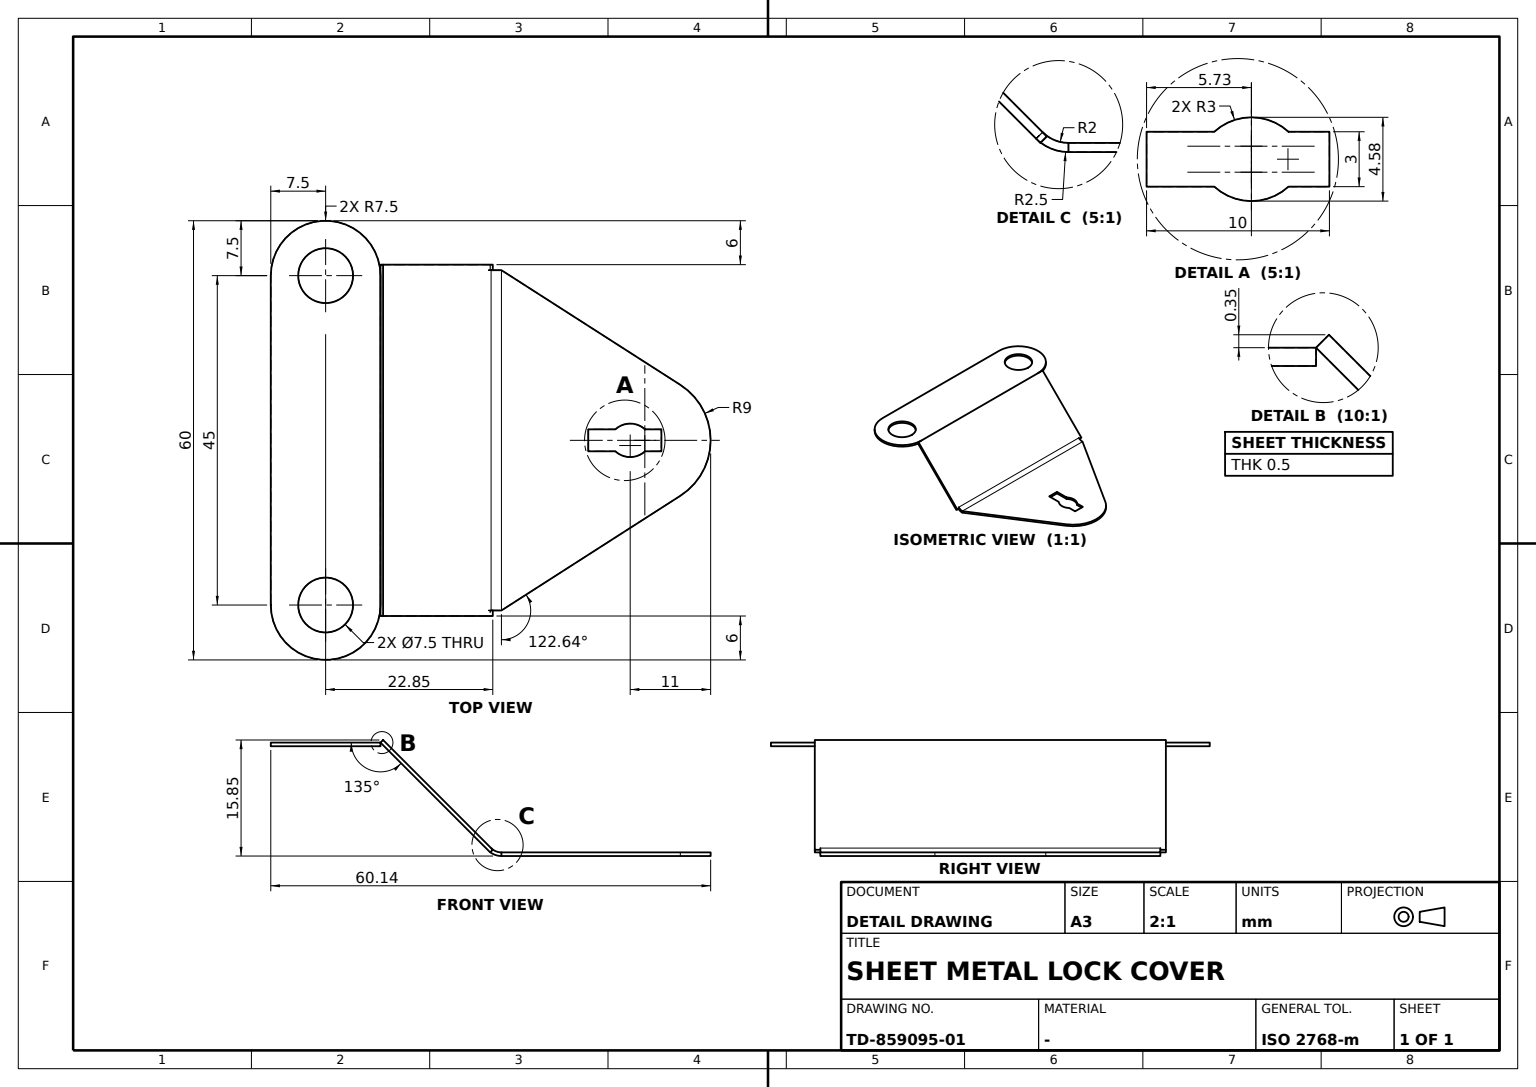
ISO-10303-21;
HEADER;
FILE_DESCRIPTION((''),'2;1');
FILE_NAME('','',(''),(''),'','','');
FILE_SCHEMA(('AUTOMOTIVE_DESIGN'));
ENDSEC;
DATA;
#1=APPLICATION_CONTEXT('');
#2=PRODUCT_CONTEXT('',#1,'mechanical');
#3=PRODUCT('','','',(#2));
#4=PRODUCT_DEFINITION_FORMATION('','',#3);
#5=PRODUCT_DEFINITION_CONTEXT('',#1,'design');
#6=PRODUCT_DEFINITION('','',#4,#5);
#7=PRODUCT_DEFINITION_SHAPE('','',#6);
#8=(LENGTH_UNIT()NAMED_UNIT(*)SI_UNIT(.MILLI.,.METRE.));
#9=(NAMED_UNIT(*)PLANE_ANGLE_UNIT()SI_UNIT($,.RADIAN.));
#10=(NAMED_UNIT(*)SI_UNIT($,.STERADIAN.)SOLID_ANGLE_UNIT());
#11=UNCERTAINTY_MEASURE_WITH_UNIT(LENGTH_MEASURE(0.005),#8,'distance_accuracy_value','');
#12=(GEOMETRIC_REPRESENTATION_CONTEXT(3)GLOBAL_UNCERTAINTY_ASSIGNED_CONTEXT((#11))GLOBAL_UNIT_ASSIGNED_CONTEXT((#8,#9,#10))REPRESENTATION_CONTEXT('',''));
#13=CARTESIAN_POINT('',(3.75,-22.5,0.5));
#14=VERTEX_POINT('',#13);
#15=CARTESIAN_POINT('',(0.,-22.5,0.5));
#16=DIRECTION('',(0.,0.,1.));
#17=DIRECTION('',(1.,0.,0.));
#18=AXIS2_PLACEMENT_3D('',#15,#16,#17);
#19=CIRCLE('',#18,3.75);
#20=EDGE_CURVE('',#14,#14,#19,.T.);
#21=ORIENTED_EDGE('',*,*,#20,.T.);
#22=EDGE_LOOP('',(#21));
#23=FACE_BOUND('',#22,.T.);
#24=CARTESIAN_POINT('',(3.75,-22.5,0.));
#25=VERTEX_POINT('',#24);
#26=CARTESIAN_POINT('',(0.,-22.5,0.));
#27=AXIS2_PLACEMENT_3D('',#26,#16,#17);
#28=CIRCLE('',#27,3.75);
#29=EDGE_CURVE('',#25,#25,#28,.T.);
#30=ORIENTED_EDGE('',*,*,#29,.F.);
#31=EDGE_LOOP('',(#30));
#32=FACE_BOUND('',#31,.T.);
#33=DIRECTION('',(0.,1.,0.));
#34=AXIS2_PLACEMENT_3D('',#15,#16,#33);
#35=CYLINDRICAL_SURFACE('',#34,3.75);
#36=ADVANCED_FACE('',(#23,#32),#35,.F.);
#37=CARTESIAN_POINT('',(3.75,22.5,0.5));
#38=VERTEX_POINT('',#37);
#39=CARTESIAN_POINT('',(0.,22.5,0.5));
#40=AXIS2_PLACEMENT_3D('',#39,#16,#17);
#41=CIRCLE('',#40,3.75);
#42=EDGE_CURVE('',#38,#38,#41,.F.);
#43=ORIENTED_EDGE('',*,*,#42,.T.);
#44=EDGE_LOOP('',(#43));
#45=FACE_BOUND('',#44,.T.);
#46=ORIENTED_EDGE('',*,*,#20,.F.);
#47=EDGE_LOOP('',(#46));
#48=FACE_BOUND('',#47,.T.);
#49=CARTESIAN_POINT('',(-7.5,-22.5,0.5));
#50=VERTEX_POINT('',#49);
#51=CARTESIAN_POINT('',(-7.5,22.5,0.5));
#52=VERTEX_POINT('',#51);
#53=VECTOR('',#33,1000.);
#54=LINE('',#51,#53);
#55=EDGE_CURVE('',#50,#52,#54,.T.);
#56=ORIENTED_EDGE('',*,*,#55,.F.);
#57=CARTESIAN_POINT('',(7.5,-22.5,0.5));
#58=VERTEX_POINT('',#57);
#59=CIRCLE('',#18,7.5);
#60=EDGE_CURVE('',#50,#58,#59,.T.);
#61=ORIENTED_EDGE('',*,*,#60,.T.);
#62=CARTESIAN_POINT('',(7.5,22.5,0.5));
#63=VERTEX_POINT('',#62);
#64=DIRECTION('',(0.,-1.,0.));
#65=VECTOR('',#64,1000.);
#66=LINE('',#57,#65);
#67=EDGE_CURVE('',#63,#58,#66,.T.);
#68=ORIENTED_EDGE('',*,*,#67,.F.);
#69=CIRCLE('',#40,7.5);
#70=EDGE_CURVE('',#63,#52,#69,.T.);
#71=ORIENTED_EDGE('',*,*,#70,.T.);
#72=EDGE_LOOP('',(#56,#61,#68,#71));
#73=FACE_BOUND('',#72,.T.);
#74=CARTESIAN_POINT('',(0.,0.,0.5));
#75=AXIS2_PLACEMENT_3D('',#74,#16,#33);
#76=PLANE('',#75);
#77=ADVANCED_FACE('',(#45,#48,#73),#76,.T.);
#78=ORIENTED_EDGE('',*,*,#42,.F.);
#79=EDGE_LOOP('',(#78));
#80=FACE_BOUND('',#79,.T.);
#81=CARTESIAN_POINT('',(3.75,22.5,0.));
#82=VERTEX_POINT('',#81);
#83=CARTESIAN_POINT('',(0.,22.5,0.));
#84=AXIS2_PLACEMENT_3D('',#83,#16,#17);
#85=CIRCLE('',#84,3.75);
#86=EDGE_CURVE('',#82,#82,#85,.F.);
#87=ORIENTED_EDGE('',*,*,#86,.T.);
#88=EDGE_LOOP('',(#87));
#89=FACE_BOUND('',#88,.T.);
#90=AXIS2_PLACEMENT_3D('',#39,#16,#33);
#91=CYLINDRICAL_SURFACE('',#90,3.75);
#92=ADVANCED_FACE('',(#80,#89),#91,.F.);
#93=CARTESIAN_POINT('',(-7.5,22.5,0.));
#94=VERTEX_POINT('',#93);
#95=VECTOR('',#16,1000.);
#96=LINE('',#93,#95);
#97=EDGE_CURVE('',#52,#94,#96,.F.);
#98=ORIENTED_EDGE('',*,*,#97,.F.);
#99=ORIENTED_EDGE('',*,*,#70,.F.);
#100=CARTESIAN_POINT('',(7.5,22.5,0.));
#101=VERTEX_POINT('',#100);
#102=LINE('',#100,#95);
#103=EDGE_CURVE('',#101,#63,#102,.T.);
#104=ORIENTED_EDGE('',*,*,#103,.F.);
#105=CIRCLE('',#84,7.5);
#106=EDGE_CURVE('',#101,#94,#105,.T.);
#107=ORIENTED_EDGE('',*,*,#106,.T.);
#108=EDGE_LOOP('',(#98,#99,#104,#107));
#109=FACE_BOUND('',#108,.T.);
#110=AXIS2_PLACEMENT_3D('',#83,#16,#33);
#111=CYLINDRICAL_SURFACE('',#110,7.5);
#112=ADVANCED_FACE('',(#109),#111,.T.);
#113=CARTESIAN_POINT('',(-7.5,-22.5,0.));
#114=VERTEX_POINT('',#113);
#115=CARTESIAN_POINT('',(7.5,-22.5,0.));
#116=VERTEX_POINT('',#115);
#117=CIRCLE('',#27,7.5);
#118=EDGE_CURVE('',#114,#116,#117,.T.);
#119=ORIENTED_EDGE('',*,*,#118,.T.);
#120=LINE('',#115,#95);
#121=EDGE_CURVE('',#116,#58,#120,.T.);
#122=ORIENTED_EDGE('',*,*,#121,.T.);
#123=ORIENTED_EDGE('',*,*,#60,.F.);
#124=LINE('',#113,#95);
#125=EDGE_CURVE('',#114,#50,#124,.T.);
#126=ORIENTED_EDGE('',*,*,#125,.F.);
#127=EDGE_LOOP('',(#119,#122,#123,#126));
#128=FACE_BOUND('',#127,.T.);
#129=AXIS2_PLACEMENT_3D('',#26,#16,#33);
#130=CYLINDRICAL_SURFACE('',#129,7.5);
#131=ADVANCED_FACE('',(#128),#130,.T.);
#132=ORIENTED_EDGE('',*,*,#103,.T.);
#133=ORIENTED_EDGE('',*,*,#67,.T.);
#134=ORIENTED_EDGE('',*,*,#121,.F.);
#135=LINE('',#115,#65);
#136=EDGE_CURVE('',#101,#116,#135,.T.);
#137=ORIENTED_EDGE('',*,*,#136,.F.);
#138=EDGE_LOOP('',(#132,#133,#134,#137));
#139=FACE_BOUND('',#138,.T.);
#140=AXIS2_PLACEMENT_3D('',#115,#17,#33);
#141=PLANE('',#140);
#142=ADVANCED_FACE('',(#139),#141,.T.);
#143=ORIENTED_EDGE('',*,*,#97,.T.);
#144=LINE('',#93,#53);
#145=EDGE_CURVE('',#114,#94,#144,.T.);
#146=ORIENTED_EDGE('',*,*,#145,.F.);
#147=ORIENTED_EDGE('',*,*,#125,.T.);
#148=ORIENTED_EDGE('',*,*,#55,.T.);
#149=EDGE_LOOP('',(#143,#146,#147,#148));
#150=FACE_BOUND('',#149,.T.);
#151=DIRECTION('',(-1.,0.,0.));
#152=AXIS2_PLACEMENT_3D('',#93,#151,#64);
#153=PLANE('',#152);
#154=ADVANCED_FACE('',(#150),#153,.T.);
#155=ORIENTED_EDGE('',*,*,#86,.F.);
#156=EDGE_LOOP('',(#155));
#157=FACE_BOUND('',#156,.T.);
#158=ORIENTED_EDGE('',*,*,#29,.T.);
#159=EDGE_LOOP('',(#158));
#160=FACE_BOUND('',#159,.T.);
#161=ORIENTED_EDGE('',*,*,#106,.F.);
#162=ORIENTED_EDGE('',*,*,#136,.T.);
#163=ORIENTED_EDGE('',*,*,#118,.F.);
#164=ORIENTED_EDGE('',*,*,#145,.T.);
#165=EDGE_LOOP('',(#161,#162,#163,#164));
#166=FACE_BOUND('',#165,.T.);
#167=CARTESIAN_POINT('',(0.,0.,0.));
#168=AXIS2_PLACEMENT_3D('',#167,#16,#33);
#169=PLANE('',#168);
#170=ADVANCED_FACE('',(#157,#160,#166),#169,.F.);
#171=CLOSED_SHELL('',(#36,#77,#92,#112,#131,#142,#154,#170));
#172=MANIFOLD_SOLID_BREP('',#171);
#173=CARTESIAN_POINT('',(48.493351,7.578879,-15.));
#174=VERTEX_POINT('',#173);
#175=CARTESIAN_POINT('',(48.493351,7.578879,-14.5));
#176=VERTEX_POINT('',#175);
#177=LINE('',#173,#95);
#178=EDGE_CURVE('',#174,#176,#177,.T.);
#179=ORIENTED_EDGE('',*,*,#178,.F.);
#180=CARTESIAN_POINT('',(24.035534,23.242995,-15.));
#181=VERTEX_POINT('',#180);
#182=CARTESIAN_POINT('',(17.547395,27.398352,-15.));
#183=DIRECTION('',(-0.84209762,0.539325133,0.));
#184=VECTOR('',#183,1000.);
#185=LINE('',#182,#184);
#186=EDGE_CURVE('',#174,#181,#185,.T.);
#187=ORIENTED_EDGE('',*,*,#186,.T.);
#188=CARTESIAN_POINT('',(24.035534,23.242995,-14.5));
#189=VERTEX_POINT('',#188);
#190=LINE('',#180,#95);
#191=EDGE_CURVE('',#181,#189,#190,.T.);
#192=ORIENTED_EDGE('',*,*,#191,.T.);
#193=CARTESIAN_POINT('',(17.547395,27.398352,-14.5));
#194=LINE('',#193,#184);
#195=EDGE_CURVE('',#176,#189,#194,.T.);
#196=ORIENTED_EDGE('',*,*,#195,.F.);
#197=EDGE_LOOP('',(#179,#187,#192,#196));
#198=FACE_BOUND('',#197,.T.);
#199=DIRECTION('',(0.539325133,0.84209762,0.));
#200=AXIS2_PLACEMENT_3D('',#173,#199,#183);
#201=PLANE('',#200);
#202=ADVANCED_FACE('',(#198),#201,.T.);
#203=CARTESIAN_POINT('',(39.611252,-1.5,-15.));
#204=VERTEX_POINT('',#203);
#205=CARTESIAN_POINT('',(39.611252,-1.5,-14.5));
#206=VERTEX_POINT('',#205);
#207=LINE('',#203,#95);
#208=EDGE_CURVE('',#204,#206,#207,.T.);
#209=ORIENTED_EDGE('',*,*,#208,.T.);
#210=CARTESIAN_POINT('',(43.667597,-1.5,-14.5));
#211=VERTEX_POINT('',#210);
#212=CARTESIAN_POINT('',(41.639425,0.710547,-14.5));
#213=AXIS2_PLACEMENT_3D('',#212,#16,#17);
#214=CIRCLE('',#213,3.);
#215=EDGE_CURVE('',#211,#206,#214,.F.);
#216=ORIENTED_EDGE('',*,*,#215,.F.);
#217=CARTESIAN_POINT('',(43.667597,-1.5,-15.));
#218=VERTEX_POINT('',#217);
#219=LINE('',#217,#95);
#220=EDGE_CURVE('',#218,#211,#219,.T.);
#221=ORIENTED_EDGE('',*,*,#220,.F.);
#222=CARTESIAN_POINT('',(41.639425,0.710547,-15.));
#223=AXIS2_PLACEMENT_3D('',#222,#16,#17);
#224=CIRCLE('',#223,3.);
#225=EDGE_CURVE('',#218,#204,#224,.F.);
#226=ORIENTED_EDGE('',*,*,#225,.T.);
#227=EDGE_LOOP('',(#209,#216,#221,#226));
#228=FACE_BOUND('',#227,.T.);
#229=AXIS2_PLACEMENT_3D('',#212,#16,#33);
#230=CYLINDRICAL_SURFACE('',#229,3.);
#231=ADVANCED_FACE('',(#228),#230,.F.);
#232=CARTESIAN_POINT('',(39.611252,1.5,-14.5));
#233=VERTEX_POINT('',#232);
#234=CARTESIAN_POINT('',(35.906857,1.5,-14.5));
#235=VERTEX_POINT('',#234);
#236=CARTESIAN_POINT('',(44.787227,1.5,-14.5));
#237=VECTOR('',#151,1000.);
#238=LINE('',#236,#237);
#239=EDGE_CURVE('',#233,#235,#238,.T.);
#240=ORIENTED_EDGE('',*,*,#239,.T.);
#241=CARTESIAN_POINT('',(35.906857,1.5,-15.));
#242=VERTEX_POINT('',#241);
#243=LINE('',#234,#95);
#244=EDGE_CURVE('',#242,#235,#243,.T.);
#245=ORIENTED_EDGE('',*,*,#244,.F.);
#246=CARTESIAN_POINT('',(39.611252,1.5,-15.));
#247=VERTEX_POINT('',#246);
#248=CARTESIAN_POINT('',(44.787227,1.5,-15.));
#249=LINE('',#248,#237);
#250=EDGE_CURVE('',#247,#242,#249,.T.);
#251=ORIENTED_EDGE('',*,*,#250,.F.);
#252=LINE('',#246,#95);
#253=EDGE_CURVE('',#247,#233,#252,.T.);
#254=ORIENTED_EDGE('',*,*,#253,.T.);
#255=EDGE_LOOP('',(#240,#245,#251,#254));
#256=FACE_BOUND('',#255,.T.);
#257=AXIS2_PLACEMENT_3D('',#236,#64,#17);
#258=PLANE('',#257);
#259=ADVANCED_FACE('',(#256),#258,.T.);
#260=CARTESIAN_POINT('',(24.035534,-23.242995,-14.5));
#261=VERTEX_POINT('',#260);
#262=CARTESIAN_POINT('',(48.493351,-7.578879,-14.5));
#263=VERTEX_POINT('',#262);
#264=CARTESIAN_POINT('',(17.547395,-27.398352,-14.5));
#265=DIRECTION('',(0.84209762,0.539325133,0.));
#266=VECTOR('',#265,1000.);
#267=LINE('',#264,#266);
#268=EDGE_CURVE('',#261,#263,#267,.T.);
#269=ORIENTED_EDGE('',*,*,#268,.T.);
#270=CARTESIAN_POINT('',(43.639425,0.,-14.5));
#271=AXIS2_PLACEMENT_3D('',#270,#16,#17);
#272=CIRCLE('',#271,9.);
#273=EDGE_CURVE('',#263,#176,#272,.T.);
#274=ORIENTED_EDGE('',*,*,#273,.T.);
#275=ORIENTED_EDGE('',*,*,#195,.T.);
#276=CARTESIAN_POINT('',(24.035534,0.,-14.5));
#277=LINE('',#276,#65);
#278=EDGE_CURVE('',#189,#261,#277,.T.);
#279=ORIENTED_EDGE('',*,*,#278,.T.);
#280=EDGE_LOOP('',(#269,#274,#275,#279));
#281=FACE_BOUND('',#280,.T.);
#282=ORIENTED_EDGE('',*,*,#239,.F.);
#283=CARTESIAN_POINT('',(43.667597,1.5,-14.5));
#284=VERTEX_POINT('',#283);
#285=CARTESIAN_POINT('',(41.639425,-0.710547,-14.5));
#286=AXIS2_PLACEMENT_3D('',#285,#16,#17);
#287=CIRCLE('',#286,3.);
#288=EDGE_CURVE('',#233,#284,#287,.F.);
#289=ORIENTED_EDGE('',*,*,#288,.T.);
#290=CARTESIAN_POINT('',(45.906857,1.5,-14.5));
#291=VERTEX_POINT('',#290);
#292=CARTESIAN_POINT('',(0.,1.5,-14.5));
#293=VECTOR('',#17,1000.);
#294=LINE('',#292,#293);
#295=EDGE_CURVE('',#284,#291,#294,.T.);
#296=ORIENTED_EDGE('',*,*,#295,.T.);
#297=CARTESIAN_POINT('',(45.906857,-1.5,-14.5));
#298=VERTEX_POINT('',#297);
#299=CARTESIAN_POINT('',(45.906857,0.,-14.5));
#300=LINE('',#299,#65);
#301=EDGE_CURVE('',#291,#298,#300,.T.);
#302=ORIENTED_EDGE('',*,*,#301,.T.);
#303=CARTESIAN_POINT('',(44.787227,-1.5,-14.5));
#304=LINE('',#303,#237);
#305=EDGE_CURVE('',#298,#211,#304,.T.);
#306=ORIENTED_EDGE('',*,*,#305,.T.);
#307=ORIENTED_EDGE('',*,*,#215,.T.);
#308=CARTESIAN_POINT('',(35.906857,-1.5,-14.5));
#309=VERTEX_POINT('',#308);
#310=EDGE_CURVE('',#206,#309,#304,.T.);
#311=ORIENTED_EDGE('',*,*,#310,.T.);
#312=CARTESIAN_POINT('',(35.906857,0.,-14.5));
#313=LINE('',#312,#53);
#314=EDGE_CURVE('',#309,#235,#313,.T.);
#315=ORIENTED_EDGE('',*,*,#314,.T.);
#316=EDGE_LOOP('',(#282,#289,#296,#302,#306,#307,#311,#315));
#317=FACE_BOUND('',#316,.T.);
#318=CARTESIAN_POINT('',(0.,0.,-14.5));
#319=AXIS2_PLACEMENT_3D('',#318,#16,#33);
#320=PLANE('',#319);
#321=ADVANCED_FACE('',(#281,#317),#320,.T.);
#322=ORIENTED_EDGE('',*,*,#253,.F.);
#323=CARTESIAN_POINT('',(43.667597,1.5,-15.));
#324=VERTEX_POINT('',#323);
#325=CARTESIAN_POINT('',(41.639425,-0.710547,-15.));
#326=AXIS2_PLACEMENT_3D('',#325,#16,#17);
#327=CIRCLE('',#326,3.);
#328=EDGE_CURVE('',#247,#324,#327,.F.);
#329=ORIENTED_EDGE('',*,*,#328,.T.);
#330=LINE('',#323,#95);
#331=EDGE_CURVE('',#324,#284,#330,.T.);
#332=ORIENTED_EDGE('',*,*,#331,.T.);
#333=ORIENTED_EDGE('',*,*,#288,.F.);
#334=EDGE_LOOP('',(#322,#329,#332,#333));
#335=FACE_BOUND('',#334,.T.);
#336=AXIS2_PLACEMENT_3D('',#285,#16,#33);
#337=CYLINDRICAL_SURFACE('',#336,3.);
#338=ADVANCED_FACE('',(#335),#337,.F.);
#339=CARTESIAN_POINT('',(7.5,-24.,0.5));
#340=VERTEX_POINT('',#339);
#341=CARTESIAN_POINT('',(22.5,-24.,-14.5));
#342=VERTEX_POINT('',#341);
#343=CARTESIAN_POINT('',(15.,-24.,-7.));
#344=DIRECTION('',(0.707106781,0.,-0.707106781));
#345=VECTOR('',#344,1000.);
#346=LINE('',#343,#345);
#347=EDGE_CURVE('',#340,#342,#346,.T.);
#348=ORIENTED_EDGE('',*,*,#347,.T.);
#349=CARTESIAN_POINT('',(22.853553,-24.,-14.146447));
#350=VERTEX_POINT('',#349);
#351=CARTESIAN_POINT('',(22.676777,-24.,-14.323223));
#352=DIRECTION('',(-0.707106781,0.,-0.707106781));
#353=VECTOR('',#352,1000.);
#354=LINE('',#351,#353);
#355=EDGE_CURVE('',#350,#342,#354,.T.);
#356=ORIENTED_EDGE('',*,*,#355,.F.);
#357=CARTESIAN_POINT('',(7.853553,-24.,0.853553));
#358=VERTEX_POINT('',#357);
#359=CARTESIAN_POINT('',(15.353553,-24.,-6.646447));
#360=LINE('',#359,#345);
#361=EDGE_CURVE('',#358,#350,#360,.T.);
#362=ORIENTED_EDGE('',*,*,#361,.F.);
#363=CARTESIAN_POINT('',(7.676777,-24.,0.676777));
#364=LINE('',#363,#353);
#365=EDGE_CURVE('',#358,#340,#364,.T.);
#366=ORIENTED_EDGE('',*,*,#365,.T.);
#367=EDGE_LOOP('',(#348,#356,#362,#366));
#368=FACE_BOUND('',#367,.T.);
#369=CARTESIAN_POINT('',(15.176777,-24.,-6.823223));
#370=AXIS2_PLACEMENT_3D('',#369,#33,#17);
#371=PLANE('',#370);
#372=ADVANCED_FACE('',(#368),#371,.F.);
#373=CARTESIAN_POINT('',(24.035534,-23.242995,-15.));
#374=VERTEX_POINT('',#373);
#375=LINE('',#373,#95);
#376=EDGE_CURVE('',#374,#261,#375,.T.);
#377=ORIENTED_EDGE('',*,*,#376,.F.);
#378=CARTESIAN_POINT('',(48.493351,-7.578879,-15.));
#379=VERTEX_POINT('',#378);
#380=CARTESIAN_POINT('',(17.547395,-27.398352,-15.));
#381=LINE('',#380,#266);
#382=EDGE_CURVE('',#374,#379,#381,.T.);
#383=ORIENTED_EDGE('',*,*,#382,.T.);
#384=LINE('',#378,#95);
#385=EDGE_CURVE('',#379,#263,#384,.T.);
#386=ORIENTED_EDGE('',*,*,#385,.T.);
#387=ORIENTED_EDGE('',*,*,#268,.F.);
#388=EDGE_LOOP('',(#377,#383,#386,#387));
#389=FACE_BOUND('',#388,.T.);
#390=CARTESIAN_POINT('',(22.853553,-24.,-15.));
#391=DIRECTION('',(0.539325133,-0.84209762,0.));
#392=AXIS2_PLACEMENT_3D('',#390,#391,#265);
#393=PLANE('',#392);
#394=ADVANCED_FACE('',(#389),#393,.T.);
#395=CARTESIAN_POINT('',(22.267767,-23.242995,-14.267767));
#396=VERTEX_POINT('',#395);
#397=CARTESIAN_POINT('',(22.62132,-23.242995,-13.914214));
#398=VERTEX_POINT('',#397);
#399=DIRECTION('',(0.707106781,0.,0.707106781));
#400=VECTOR('',#399,1000.);
#401=LINE('',#395,#400);
#402=EDGE_CURVE('',#396,#398,#401,.T.);
#403=ORIENTED_EDGE('',*,*,#402,.F.);
#404=CARTESIAN_POINT('',(24.035534,-23.242995,-12.5));
#405=DIRECTION('',(0.,0.,-1.));
#406=AXIS2_PLACEMENT_3D('',#404,#64,#405);
#407=CIRCLE('',#406,2.5);
#408=EDGE_CURVE('',#396,#374,#407,.T.);
#409=ORIENTED_EDGE('',*,*,#408,.T.);
#410=ORIENTED_EDGE('',*,*,#376,.T.);
#411=CIRCLE('',#406,2.);
#412=EDGE_CURVE('',#398,#261,#411,.T.);
#413=ORIENTED_EDGE('',*,*,#412,.F.);
#414=EDGE_LOOP('',(#403,#409,#410,#413));
#415=FACE_BOUND('',#414,.T.);
#416=CARTESIAN_POINT('',(23.878454,-23.242995,-14.5));
#417=CARTESIAN_POINT('',(23.839184,-23.242995,-15.));
#418=CARTESIAN_POINT('',(23.721375,-23.242995,-14.484579));
#419=CARTESIAN_POINT('',(23.642835,-23.242995,-14.980723));
#420=CARTESIAN_POINT('',(23.566314,-23.242995,-14.453735));
#421=CARTESIAN_POINT('',(23.449009,-23.242995,-14.942169));
#422=CARTESIAN_POINT('',(23.264266,-23.242995,-14.362006));
#423=CARTESIAN_POINT('',(23.071449,-23.242995,-14.827508));
#424=CARTESIAN_POINT('',(22.985823,-23.242995,-14.213288));
#425=CARTESIAN_POINT('',(22.723396,-23.242995,-14.64161));
#426=CARTESIAN_POINT('',(22.854369,-23.242995,-14.125453));
#427=CARTESIAN_POINT('',(22.559078,-23.242995,-14.531817));
#428=CARTESIAN_POINT('',(22.732392,-23.242995,-14.025286));
#429=CARTESIAN_POINT('',(22.406607,-23.242995,-14.406607));
#430=B_SPLINE_SURFACE_WITH_KNOTS('',5,1,((#260,#373),(#416,#417),(#418,#419),(#420,#421),(#422,#423),(#424,#425),(#426,#427),(#428,#429),(#397,#395)),.RULED_SURF.,.F.,.F.,.F.,(6,3,6),(2,2),(0.,0.00185,0.0037),(0.,0.00049),.UNSPECIFIED.);
#431=ADVANCED_FACE('',(#415),#430,.T.);
#432=ORIENTED_EDGE('',*,*,#191,.F.);
#433=CARTESIAN_POINT('',(22.267767,23.242995,-14.267767));
#434=VERTEX_POINT('',#433);
#435=CARTESIAN_POINT('',(24.035534,23.242995,-12.5));
#436=AXIS2_PLACEMENT_3D('',#435,#64,#405);
#437=CIRCLE('',#436,2.5);
#438=EDGE_CURVE('',#434,#181,#437,.T.);
#439=ORIENTED_EDGE('',*,*,#438,.F.);
#440=CARTESIAN_POINT('',(22.62132,23.242995,-13.914214));
#441=VERTEX_POINT('',#440);
#442=LINE('',#440,#353);
#443=EDGE_CURVE('',#434,#441,#442,.F.);
#444=ORIENTED_EDGE('',*,*,#443,.T.);
#445=CIRCLE('',#436,2.);
#446=EDGE_CURVE('',#441,#189,#445,.T.);
#447=ORIENTED_EDGE('',*,*,#446,.T.);
#448=EDGE_LOOP('',(#432,#439,#444,#447));
#449=FACE_BOUND('',#448,.T.);
#450=CARTESIAN_POINT('',(23.878454,23.242995,-14.5));
#451=CARTESIAN_POINT('',(23.839184,23.242995,-15.));
#452=CARTESIAN_POINT('',(23.721375,23.242995,-14.484579));
#453=CARTESIAN_POINT('',(23.642835,23.242995,-14.980723));
#454=CARTESIAN_POINT('',(23.566314,23.242995,-14.453735));
#455=CARTESIAN_POINT('',(23.449009,23.242995,-14.942169));
#456=CARTESIAN_POINT('',(23.264266,23.242995,-14.362006));
#457=CARTESIAN_POINT('',(23.071449,23.242995,-14.827508));
#458=CARTESIAN_POINT('',(22.985823,23.242995,-14.213288));
#459=CARTESIAN_POINT('',(22.723396,23.242995,-14.64161));
#460=CARTESIAN_POINT('',(22.854369,23.242995,-14.125453));
#461=CARTESIAN_POINT('',(22.559078,23.242995,-14.531817));
#462=CARTESIAN_POINT('',(22.732392,23.242995,-14.025286));
#463=CARTESIAN_POINT('',(22.406607,23.242995,-14.406607));
#464=B_SPLINE_SURFACE_WITH_KNOTS('',5,1,((#188,#180),(#450,#451),(#452,#453),(#454,#455),(#456,#457),(#458,#459),(#460,#461),(#462,#463),(#440,#433)),.RULED_SURF.,.F.,.F.,.F.,(6,3,6),(2,2),(0.,0.00185,0.0037),(0.,0.00049),.UNSPECIFIED.);
#465=ADVANCED_FACE('',(#449),#464,.F.);
#466=CARTESIAN_POINT('',(22.62132,0.,-13.914214));
#467=LINE('',#466,#65);
#468=EDGE_CURVE('',#441,#398,#467,.T.);
#469=ORIENTED_EDGE('',*,*,#468,.T.);
#470=ORIENTED_EDGE('',*,*,#412,.T.);
#471=ORIENTED_EDGE('',*,*,#278,.F.);
#472=ORIENTED_EDGE('',*,*,#446,.F.);
#473=EDGE_LOOP('',(#469,#470,#471,#472));
#474=FACE_BOUND('',#473,.T.);
#475=CARTESIAN_POINT('',(24.035534,0.,-12.5));
#476=AXIS2_PLACEMENT_3D('',#475,#64,#405);
#477=CYLINDRICAL_SURFACE('',#476,2.);
#478=ADVANCED_FACE('',(#474),#477,.F.);
#479=CARTESIAN_POINT('',(45.906857,-1.5,-15.));
#480=VERTEX_POINT('',#479);
#481=LINE('',#297,#95);
#482=EDGE_CURVE('',#480,#298,#481,.T.);
#483=ORIENTED_EDGE('',*,*,#482,.T.);
#484=ORIENTED_EDGE('',*,*,#301,.F.);
#485=CARTESIAN_POINT('',(45.906857,1.5,-15.));
#486=VERTEX_POINT('',#485);
#487=LINE('',#290,#95);
#488=EDGE_CURVE('',#486,#291,#487,.T.);
#489=ORIENTED_EDGE('',*,*,#488,.F.);
#490=CARTESIAN_POINT('',(45.906857,0.,-15.));
#491=LINE('',#490,#65);
#492=EDGE_CURVE('',#486,#480,#491,.T.);
#493=ORIENTED_EDGE('',*,*,#492,.T.);
#494=EDGE_LOOP('',(#483,#484,#489,#493));
#495=FACE_BOUND('',#494,.T.);
#496=AXIS2_PLACEMENT_3D('',#299,#151,#33);
#497=PLANE('',#496);
#498=ADVANCED_FACE('',(#495),#497,.T.);
#499=ORIENTED_EDGE('',*,*,#438,.T.);
#500=CARTESIAN_POINT('',(24.035534,0.,-15.));
#501=LINE('',#500,#65);
#502=EDGE_CURVE('',#181,#374,#501,.T.);
#503=ORIENTED_EDGE('',*,*,#502,.T.);
#504=ORIENTED_EDGE('',*,*,#408,.F.);
#505=CARTESIAN_POINT('',(22.267767,0.,-14.267767));
#506=LINE('',#505,#65);
#507=EDGE_CURVE('',#434,#396,#506,.T.);
#508=ORIENTED_EDGE('',*,*,#507,.F.);
#509=EDGE_LOOP('',(#499,#503,#504,#508));
#510=FACE_BOUND('',#509,.T.);
#511=CYLINDRICAL_SURFACE('',#476,2.5);
#512=ADVANCED_FACE('',(#510),#511,.T.);
#513=CARTESIAN_POINT('',(7.5,24.,0.5));
#514=VERTEX_POINT('',#513);
#515=CARTESIAN_POINT('',(7.5,0.,0.5));
#516=LINE('',#515,#53);
#517=EDGE_CURVE('',#340,#514,#516,.T.);
#518=ORIENTED_EDGE('',*,*,#517,.T.);
#519=CARTESIAN_POINT('',(22.5,24.,-14.5));
#520=VERTEX_POINT('',#519);
#521=CARTESIAN_POINT('',(15.,24.,-7.));
#522=LINE('',#521,#345);
#523=EDGE_CURVE('',#514,#520,#522,.T.);
#524=ORIENTED_EDGE('',*,*,#523,.T.);
#525=CARTESIAN_POINT('',(22.5,23.242995,-14.5));
#526=VERTEX_POINT('',#525);
#527=CARTESIAN_POINT('',(22.5,0.,-14.5));
#528=LINE('',#527,#53);
#529=EDGE_CURVE('',#526,#520,#528,.T.);
#530=ORIENTED_EDGE('',*,*,#529,.F.);
#531=CARTESIAN_POINT('',(22.383883,23.242995,-14.383883));
#532=LINE('',#531,#345);
#533=EDGE_CURVE('',#434,#526,#532,.T.);
#534=ORIENTED_EDGE('',*,*,#533,.F.);
#535=ORIENTED_EDGE('',*,*,#507,.T.);
#536=CARTESIAN_POINT('',(22.5,-23.242995,-14.5));
#537=VERTEX_POINT('',#536);
#538=CARTESIAN_POINT('',(7.5,-23.242995,0.5));
#539=DIRECTION('',(-0.707106781,0.,0.707106781));
#540=VECTOR('',#539,1000.);
#541=LINE('',#538,#540);
#542=EDGE_CURVE('',#537,#396,#541,.T.);
#543=ORIENTED_EDGE('',*,*,#542,.F.);
#544=EDGE_CURVE('',#342,#537,#528,.T.);
#545=ORIENTED_EDGE('',*,*,#544,.F.);
#546=ORIENTED_EDGE('',*,*,#347,.F.);
#547=EDGE_LOOP('',(#518,#524,#530,#534,#535,#543,#545,#546));
#548=FACE_BOUND('',#547,.T.);
#549=AXIS2_PLACEMENT_3D('',#515,#399,#344);
#550=PLANE('',#549);
#551=ADVANCED_FACE('',(#548),#550,.F.);
#552=ORIENTED_EDGE('',*,*,#443,.F.);
#553=ORIENTED_EDGE('',*,*,#533,.T.);
#554=CARTESIAN_POINT('',(22.853553,23.242995,-14.146447));
#555=VERTEX_POINT('',#554);
#556=LINE('',#525,#400);
#557=EDGE_CURVE('',#526,#555,#556,.T.);
#558=ORIENTED_EDGE('',*,*,#557,.T.);
#559=CARTESIAN_POINT('',(22.737437,23.242995,-14.03033));
#560=LINE('',#559,#345);
#561=EDGE_CURVE('',#441,#555,#560,.T.);
#562=ORIENTED_EDGE('',*,*,#561,.F.);
#563=EDGE_LOOP('',(#552,#553,#558,#562));
#564=FACE_BOUND('',#563,.T.);
#565=AXIS2_PLACEMENT_3D('',#531,#33,#17);
#566=PLANE('',#565);
#567=ADVANCED_FACE('',(#564),#566,.F.);
#568=ORIENTED_EDGE('',*,*,#523,.F.);
#569=CARTESIAN_POINT('',(7.853553,24.,0.853553));
#570=VERTEX_POINT('',#569);
#571=CARTESIAN_POINT('',(7.676777,24.,0.676777));
#572=LINE('',#571,#353);
#573=EDGE_CURVE('',#570,#514,#572,.T.);
#574=ORIENTED_EDGE('',*,*,#573,.F.);
#575=CARTESIAN_POINT('',(22.853553,24.,-14.146447));
#576=VERTEX_POINT('',#575);
#577=CARTESIAN_POINT('',(15.353553,24.,-6.646447));
#578=LINE('',#577,#345);
#579=EDGE_CURVE('',#570,#576,#578,.T.);
#580=ORIENTED_EDGE('',*,*,#579,.T.);
#581=CARTESIAN_POINT('',(22.676777,24.,-14.323223));
#582=LINE('',#581,#353);
#583=EDGE_CURVE('',#576,#520,#582,.T.);
#584=ORIENTED_EDGE('',*,*,#583,.T.);
#585=EDGE_LOOP('',(#568,#574,#580,#584));
#586=FACE_BOUND('',#585,.T.);
#587=CARTESIAN_POINT('',(15.176777,24.,-6.823223));
#588=AXIS2_PLACEMENT_3D('',#587,#33,#17);
#589=PLANE('',#588);
#590=ADVANCED_FACE('',(#586),#589,.T.);
#591=ORIENTED_EDGE('',*,*,#557,.F.);
#592=ORIENTED_EDGE('',*,*,#529,.T.);
#593=ORIENTED_EDGE('',*,*,#583,.F.);
#594=CARTESIAN_POINT('',(22.853553,0.,-14.146447));
#595=LINE('',#594,#53);
#596=EDGE_CURVE('',#555,#576,#595,.T.);
#597=ORIENTED_EDGE('',*,*,#596,.F.);
#598=EDGE_LOOP('',(#591,#592,#593,#597));
#599=FACE_BOUND('',#598,.T.);
#600=CARTESIAN_POINT('',(22.676777,0.,-14.323223));
#601=AXIS2_PLACEMENT_3D('',#600,#539,#399);
#602=PLANE('',#601);
#603=ADVANCED_FACE('',(#599),#602,.F.);
#604=CARTESIAN_POINT('',(44.787227,-1.5,-15.));
#605=LINE('',#604,#237);
#606=EDGE_CURVE('',#480,#218,#605,.T.);
#607=ORIENTED_EDGE('',*,*,#606,.F.);
#608=ORIENTED_EDGE('',*,*,#492,.F.);
#609=CARTESIAN_POINT('',(0.,1.5,-15.));
#610=LINE('',#609,#293);
#611=EDGE_CURVE('',#324,#486,#610,.T.);
#612=ORIENTED_EDGE('',*,*,#611,.F.);
#613=ORIENTED_EDGE('',*,*,#328,.F.);
#614=ORIENTED_EDGE('',*,*,#250,.T.);
#615=CARTESIAN_POINT('',(35.906857,-1.5,-15.));
#616=VERTEX_POINT('',#615);
#617=CARTESIAN_POINT('',(35.906857,0.,-15.));
#618=LINE('',#617,#53);
#619=EDGE_CURVE('',#616,#242,#618,.T.);
#620=ORIENTED_EDGE('',*,*,#619,.F.);
#621=EDGE_CURVE('',#204,#616,#605,.T.);
#622=ORIENTED_EDGE('',*,*,#621,.F.);
#623=ORIENTED_EDGE('',*,*,#225,.F.);
#624=EDGE_LOOP('',(#607,#608,#612,#613,#614,#620,#622,#623));
#625=FACE_BOUND('',#624,.T.);
#626=ORIENTED_EDGE('',*,*,#502,.F.);
#627=ORIENTED_EDGE('',*,*,#186,.F.);
#628=CARTESIAN_POINT('',(43.639425,0.,-15.));
#629=AXIS2_PLACEMENT_3D('',#628,#16,#17);
#630=CIRCLE('',#629,9.);
#631=EDGE_CURVE('',#379,#174,#630,.T.);
#632=ORIENTED_EDGE('',*,*,#631,.F.);
#633=ORIENTED_EDGE('',*,*,#382,.F.);
#634=EDGE_LOOP('',(#626,#627,#632,#633));
#635=FACE_BOUND('',#634,.T.);
#636=CARTESIAN_POINT('',(0.,0.,-15.));
#637=AXIS2_PLACEMENT_3D('',#636,#16,#33);
#638=PLANE('',#637);
#639=ADVANCED_FACE('',(#625,#635),#638,.F.);
#640=ORIENTED_EDGE('',*,*,#314,.F.);
#641=LINE('',#308,#95);
#642=EDGE_CURVE('',#616,#309,#641,.T.);
#643=ORIENTED_EDGE('',*,*,#642,.F.);
#644=ORIENTED_EDGE('',*,*,#619,.T.);
#645=ORIENTED_EDGE('',*,*,#244,.T.);
#646=EDGE_LOOP('',(#640,#643,#644,#645));
#647=FACE_BOUND('',#646,.T.);
#648=AXIS2_PLACEMENT_3D('',#312,#17,#33);
#649=PLANE('',#648);
#650=ADVANCED_FACE('',(#647),#649,.T.);
#651=ORIENTED_EDGE('',*,*,#596,.T.);
#652=ORIENTED_EDGE('',*,*,#579,.F.);
#653=CARTESIAN_POINT('',(7.853553,0.,0.853553));
#654=LINE('',#653,#53);
#655=EDGE_CURVE('',#358,#570,#654,.T.);
#656=ORIENTED_EDGE('',*,*,#655,.F.);
#657=ORIENTED_EDGE('',*,*,#361,.T.);
#658=CARTESIAN_POINT('',(22.853553,-23.242995,-14.146447));
#659=VERTEX_POINT('',#658);
#660=EDGE_CURVE('',#350,#659,#595,.T.);
#661=ORIENTED_EDGE('',*,*,#660,.T.);
#662=CARTESIAN_POINT('',(7.853553,-23.242995,0.853553));
#663=LINE('',#662,#540);
#664=EDGE_CURVE('',#659,#398,#663,.T.);
#665=ORIENTED_EDGE('',*,*,#664,.T.);
#666=ORIENTED_EDGE('',*,*,#468,.F.);
#667=ORIENTED_EDGE('',*,*,#561,.T.);
#668=EDGE_LOOP('',(#651,#652,#656,#657,#661,#665,#666,#667));
#669=FACE_BOUND('',#668,.T.);
#670=AXIS2_PLACEMENT_3D('',#653,#399,#344);
#671=PLANE('',#670);
#672=ADVANCED_FACE('',(#669),#671,.T.);
#673=ORIENTED_EDGE('',*,*,#517,.F.);
#674=ORIENTED_EDGE('',*,*,#365,.F.);
#675=ORIENTED_EDGE('',*,*,#655,.T.);
#676=ORIENTED_EDGE('',*,*,#573,.T.);
#677=EDGE_LOOP('',(#673,#674,#675,#676));
#678=FACE_BOUND('',#677,.T.);
#679=CARTESIAN_POINT('',(7.676777,0.,0.676777));
#680=AXIS2_PLACEMENT_3D('',#679,#539,#399);
#681=PLANE('',#680);
#682=ADVANCED_FACE('',(#678),#681,.T.);
#683=ORIENTED_EDGE('',*,*,#273,.F.);
#684=ORIENTED_EDGE('',*,*,#385,.F.);
#685=ORIENTED_EDGE('',*,*,#631,.T.);
#686=ORIENTED_EDGE('',*,*,#178,.T.);
#687=EDGE_LOOP('',(#683,#684,#685,#686));
#688=FACE_BOUND('',#687,.T.);
#689=AXIS2_PLACEMENT_3D('',#628,#16,#33);
#690=CYLINDRICAL_SURFACE('',#689,9.);
#691=ADVANCED_FACE('',(#688),#690,.T.);
#692=ORIENTED_EDGE('',*,*,#542,.T.);
#693=ORIENTED_EDGE('',*,*,#402,.T.);
#694=ORIENTED_EDGE('',*,*,#664,.F.);
#695=LINE('',#536,#400);
#696=EDGE_CURVE('',#537,#659,#695,.T.);
#697=ORIENTED_EDGE('',*,*,#696,.F.);
#698=EDGE_LOOP('',(#692,#693,#694,#697));
#699=FACE_BOUND('',#698,.T.);
#700=CARTESIAN_POINT('',(22.383883,-23.242995,-14.383883));
#701=AXIS2_PLACEMENT_3D('',#700,#33,#17);
#702=PLANE('',#701);
#703=ADVANCED_FACE('',(#699),#702,.T.);
#704=ORIENTED_EDGE('',*,*,#611,.T.);
#705=ORIENTED_EDGE('',*,*,#488,.T.);
#706=ORIENTED_EDGE('',*,*,#295,.F.);
#707=ORIENTED_EDGE('',*,*,#331,.F.);
#708=EDGE_LOOP('',(#704,#705,#706,#707));
#709=FACE_BOUND('',#708,.T.);
#710=ADVANCED_FACE('',(#709),#258,.T.);
#711=ORIENTED_EDGE('',*,*,#606,.T.);
#712=ORIENTED_EDGE('',*,*,#220,.T.);
#713=ORIENTED_EDGE('',*,*,#305,.F.);
#714=ORIENTED_EDGE('',*,*,#482,.F.);
#715=EDGE_LOOP('',(#711,#712,#713,#714));
#716=FACE_BOUND('',#715,.T.);
#717=AXIS2_PLACEMENT_3D('',#303,#64,#17);
#718=PLANE('',#717);
#719=ADVANCED_FACE('',(#716),#718,.F.);
#720=ORIENTED_EDGE('',*,*,#696,.T.);
#721=ORIENTED_EDGE('',*,*,#660,.F.);
#722=ORIENTED_EDGE('',*,*,#355,.T.);
#723=ORIENTED_EDGE('',*,*,#544,.T.);
#724=EDGE_LOOP('',(#720,#721,#722,#723));
#725=FACE_BOUND('',#724,.T.);
#726=ADVANCED_FACE('',(#725),#602,.F.);
#727=ORIENTED_EDGE('',*,*,#642,.T.);
#728=ORIENTED_EDGE('',*,*,#310,.F.);
#729=ORIENTED_EDGE('',*,*,#208,.F.);
#730=ORIENTED_EDGE('',*,*,#621,.T.);
#731=EDGE_LOOP('',(#727,#728,#729,#730));
#732=FACE_BOUND('',#731,.T.);
#733=ADVANCED_FACE('',(#732),#718,.F.);
#734=CLOSED_SHELL('',(#202,#231,#259,#321,#338,#372,#394,#431,#465,#478,#498,#512,#551,#567,#590,#603,#639,#650,#672,#682,#691,#703,#710,#719,#726,#733));
#735=MANIFOLD_SOLID_BREP('',#734);
#736=ADVANCED_BREP_SHAPE_REPRESENTATION('',(#172,#735),#12);
#737=SHAPE_DEFINITION_REPRESENTATION(#7,#736);
ENDSEC;
END-ISO-10303-21;
